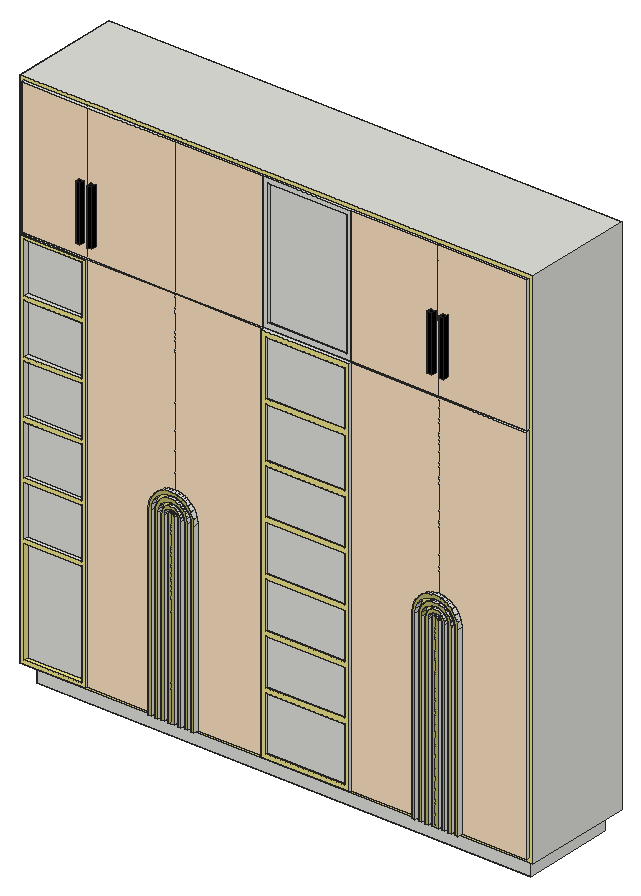
# SketchUp Ruby script. Lengths in inches.
U = 1.inch
M = Sketchup.active_model
def pt(a) = Geom::Point3d.new(a.map { |v| v * U })
def face(e, loops, mat)
  f = e.add_face(loops[0].map { |a| pt(a) })
  loops[1..].each { |l| e.add_face(l.map { |a| pt(a) }).erase! }
  f.material = f.back_material = mat if mat
  f
end
# faces: each face lists its corners as indices into pts; further lists are holes
def faces(e, pts, list, mat = nil) = list.each { |f| face(e, (f[0].is_a?(Array) ? f : [f]).map { |l| l.map { |i| pts[i] } }, mat) }
# xy, xz, yz: faces in a plane at the given z, y or x. An outline is a flat list of corners, or four numbers for a rectangle; further outlines are holes
def ring(l) = l.size == 4 ? [[l[0], l[1]], [l[2], l[1]], [l[2], l[3]], [l[0], l[3]]] : l.each_slice(2).to_a
def flat(e, list, mat, &to3) = list.each { |f| face(e, (f[0].is_a?(Array) ? f : [f]).map { |l| ring(l).map { |u, v| to3.(u, v) } }, mat) }
def xy(e, z, list, mat = nil) = flat(e, list, mat) { |x, y| [x, y, z] }
def xz(e, y, list, mat = nil) = flat(e, list, mat) { |x, z| [x, y, z] }
def yz(e, x, list, mat = nil) = flat(e, list, mat) { |y, z| [x, y, z] }
def lines(e, pts, list) = list.each { |a, b| e.add_line(pt(pts[a]), pt(pts[b])) }
# prism: a flat outline (further loops are holes) pulled along v
def prism(e, loops, v, mat = nil)
  f = face(e, loops, mat); d = Geom::Vector3d.new(v.map { |x| x * U })
  f.pushpull(f.normal.samedirection?(d) ? d.length : -d.length)
end
def box(e, o, s, mat = nil) = prism(e, [[o, [o[0] + s[0], o[1], o[2]], [o[0] + s[0], o[1] + s[1], o[2]], [o[0], o[1] + s[1], o[2]]]], [0, 0, s[2]], mat)
def at(x, y, z, deg = 0) = Geom::Transformation.translation(pt([x, y, z])) * Geom::Transformation.rotation(ORIGIN, Z_AXIS, deg.degrees)
def axes(o, x, y, z) = Geom::Transformation.new([*x, 0, *y, 0, *z, 0, *pt(o).to_a, 1])
def part(name) = M.definitions.add(name)
# library, detail: a bought-in or finely detailed component or shape, given as its bounding box
def library(name, o, s) = part(name).tap { |d| box(d.entities, o, s) }
def detail(e, o, s) = box(e.add_group.entities, o, s)
def put(e, d, t, mat = nil) = e.add_instance(d, t).tap { |i| i.material = mat if mat }
def group(e, t, mat = nil) = e.add_group.tap { |g| g.transformation = t; g.material = mat if mat }.entities
root = M.entities
M.materials.add("[0012_Bisque]").color = [255, 228, 196]
M.materials.add("[0047_Khaki]").color = [240, 230, 140]
M.materials.add("[0057_DarkKhaki]").color = [189, 183, 107]
M.materials.add("[0137_Black]").color = [0, 0, 0]
xy(root,-4,[[2,3.6,109,23.6]])
xy(root,0,[[[0,1.6,111,25.6],[2,3.6,109,23.6]]])
xy(root,0.8,[[0.8,0.6,15,1.6],[53,0.6,72,1.6]])
xy(root,0.8,[[29,0,29,1,15,1,15,1.6,34,1.6,34,0,33.29,0,33.29,1,32.57,1,32.57,0,31.86,0,31.86,1,31.14,1,31.14,0,30.43,0,30.43,1,29.71,1,29.71,0],[34,0,34,1.6,53,1.6,53,1,39,1,39,0,38.29,0,38.29,1,37.57,1,37.57,0,36.86,0,36.86,1,36.14,1,36.14,0,35.43,0,35.43,1,34.71,1,34.71,0],[86.1,0,86.1,1,72,1,72,1.6,91.1,1.6,91.1,0,90.39,0,90.39,1,89.67,1,89.67,0,88.96,0,88.96,1,88.24,1,88.24,0,87.53,0,87.53,1,86.8125,1,86.8125,0],[91.1,0,91.1,1.6,110.2,1.6,110.2,1,96.1,1,96.1,0,95.39,0,95.39,1,94.67,1,94.67,0,93.96,0,93.96,1,93.24,1,93.24,0,92.53,0,92.53,1,91.8125,1,91.8125,0]],"[0047_Khaki]")
xy(root,1.6,[[1.6,0.6,14.2,1.6]],"[0047_Khaki]")
xy(root,1.8,[[54,0.6,71,1]],"[0047_Khaki]")
xy(root,13.63,[[54,0.6,71,1]])
xy(root,14.63,[[54,0.6,71,1]],"[0047_Khaki]")
xy(root,24.2,[[1.6,0.6,14.2,1.6]])
xy(root,24.63,[[54,0.6,71,1]])
xy(root,25,[[1.6,0.6,14.2,1.6]])
xy(root,25.63,[[54,0.6,71,1]],"[0047_Khaki]")
xy(root,35.63,[[54,0.6,71,1]])
xy(root,36,[[1.6,0.6,14.2,1.6]])
xy(root,36.63,[[54,0.6,71,1]])
xy(root,36.8,[[1.6,0.6,14.2,1.6]])
xy(root,46.63,[[54,0.6,71,1]])
xy(root,47.63,[[54,0.6,71,1]])
xy(root,47.8,[[1.6,0.6,14.2,1.6]])
xy(root,48.6,[[1.6,0.6,14.2,1.6]])
xy(root,57.63,[[54,0.6,71,1]])
xy(root,58.63,[[54,0.6,71,1]])
xy(root,59.6,[[1.6,0.6,14.2,1.6]])
xy(root,60.4,[[1.6,0.6,14.2,1.6]])
xy(root,69.63,[[54,0.6,71,1]])
xy(root,70.63,[[54,0.6,71,1]])
xy(root,71.4,[[1.6,0.6,14.2,1.6]])
xy(root,72.2,[[1.6,0.6,14.2,1.6]])
xy(root,82.63,[[54,0.6,71,1]])
xy(root,83.2,[[1.6,0.6,14.2,1.6]])
xy(root,83.63,[[0.8,0.6,15,1],[53,0.6,72,0.6,72,1,110.2,1,110.2,1.6,0.8,1.6,0.8,1,53,1]])
xy(root,84,[[0.8,1,110.2,1.6],[53,1,72,1.125]])
xy(root,85,[[54,1.125,71,1.6]])
xy(root,86.77,[[13.29,0,14.29,1],[15.79,0,16.79,1]],"[0137_Black]")
xy(root,88.27,[[89.41,0,90.41,1],[91.97,0,92.97,1]],"[0137_Black]")
xy(root,98.77,[[13.29,0,14.29,1],[15.79,0,16.79,1]],"[0137_Black]")
xy(root,100.27,[[89.41,0,90.41,1],[91.97,0,92.97,1]],"[0137_Black]")
xy(root,112.2,[[54,1.125,71,1.6]])
xy(root,113.2,[[0.8,1,15,1.6],[15,1,34,1.6],[34,1,53,1.6],[72,1,91,1.6],[91,1,110.2,1.6],
  [53,1.125,72,1.6]])
xy(root,114,[[0,1.6,111,25.6]])
xz(root,0,[[29,0.8,29.71,0.8,29.71,40.8,29.86,41.91,30.29,42.94,30.43,43.125,30.97,43.83,31.14,43.96,31.86,44.51,32.57,44.81,32.89,44.94,33.29,44.99,34,45.09,34.71,44.99,35.11,44.94,35.43,44.81,36.14,44.51,36.86,43.96,37.03,43.83,37.57,43.125,37.71,42.94,38.14,41.91,38.29,40.8,38.29,0.8,39,0.8,39,40.8,38.83,42.09,38.33,43.3,38.29,43.36,37.57,44.29,37.54,44.34,36.86,44.86,36.5,45.13,36.14,45.28,35.43,45.57,35.29,45.63,34.71,45.71,34,45.8,33.29,45.71,32.71,45.63,32.57,45.57,31.86,45.28,31.5,45.13,31.14,44.86,30.46,44.34,30.43,44.29,29.71,43.36,29.67,43.3,29.17,42.09,29,40.8],[30.43,0.8,31.14,0.8,31.14,40.8,31.24,41.54,31.53,42.23,31.86,42.66,31.98,42.82,32.57,43.27,33.26,43.56,33.29,43.5625,34,43.66,34.71,43.5625,34.74,43.56,35.43,43.27,36.02,42.82,36.14,42.66,36.47,42.23,36.76,41.54,36.86,40.8,36.86,0.8,37.57,0.8,37.57,40.8,37.45,41.72,37.09,42.59,36.86,42.89,36.53,43.33,36.14,43.62,35.79,43.89,35.43,44.04,34.92,44.25,34.71,44.28,34,44.37,33.29,44.28,33.08,44.25,32.57,44.04,32.21,43.89,31.86,43.62,31.47,43.33,31.14,42.89,30.91,42.59,30.55,41.72,30.43,40.8],[31.86,0.8,32.57,0.8,32.57,40.8,32.59,41.2,32.72,41.57,32.94,41.9,33.25,42.15,33.29,42.17,33.61,42.31,34,42.36,34.39,42.31,34.71,42.17,34.75,42.15,35.06,41.9,35.28,41.57,35.41,41.2,35.43,40.8,35.43,0.8,36.14,0.8,36.14,40.8,36.07,41.35,35.86,41.87,35.52,42.32,35.43,42.38,35.07,42.66,34.71,42.8,34.55,42.87,34,42.94,33.45,42.87,33.29,42.8,32.93,42.66,32.57,42.38,32.48,42.32,32.14,41.87,31.93,41.35,31.86,40.8],[33.29,0.8,34,0.8,34,41.8,33.83,41.78,33.67,41.72,33.52,41.62,33.41,41.49,33.33,41.34,33.29,41.17],[34,0.8,34.71,0.8,34.71,41.17,34.67,41.34,34.59,41.49,34.48,41.62,34.33,41.72,34.17,41.78,34,41.8],
  [86.1,0.8,86.8125,0.8,86.8125,40.8,86.96,41.91,87.39,42.94,87.53,43.125,88.07,43.83,88.24,43.96,88.96,44.51,89.67,44.81,89.99,44.94,90.39,44.99,91.1,45.09,91.8125,44.99,92.21,44.94,92.53,44.81,93.24,44.51,93.96,43.96,94.13,43.83,94.67,43.125,94.8125,42.94,95.24,41.91,95.39,40.8,95.39,0.8,96.1,0.8,96.1,40.8,95.93,42.09,95.43,43.3,95.39,43.36,94.67,44.29,94.64,44.34,93.96,44.86,93.6,45.13,93.24,45.28,92.53,45.57,92.39,45.63,91.8125,45.71,91.1,45.8,90.39,45.71,89.81,45.63,89.67,45.57,88.96,45.28,88.6,45.13,88.24,44.86,87.5625,44.34,87.53,44.29,86.8125,43.36,86.77,43.3,86.27,42.09,86.1,40.8],[87.53,0.8,88.24,0.8,88.24,40.8,88.34,41.54,88.625,42.23,88.96,42.66,89.08,42.82,89.67,43.27,90.36,43.56,90.39,43.5625,91.1,43.66,91.8125,43.5625,91.84,43.56,92.53,43.27,93.12,42.82,93.24,42.66,93.57,42.23,93.86,41.54,93.96,40.8,93.96,0.8,94.67,0.8,94.67,40.8,94.55,41.72,94.19,42.59,93.96,42.89,93.625,43.33,93.24,43.62,92.89,43.89,92.53,44.04,92.02,44.25,91.8125,44.28,91.1,44.37,90.39,44.28,90.18,44.25,89.67,44.04,89.3125,43.89,88.96,43.62,88.57,43.33,88.24,42.89,88.01,42.59,87.65,41.72,87.53,40.8],[88.96,0.8,89.67,0.8,89.67,40.8,89.69,41.2,89.82,41.57,90.04,41.9,90.35,42.15,90.39,42.17,90.71,42.31,91.1,42.36,91.49,42.31,91.8125,42.17,91.85,42.15,92.16,41.9,92.38,41.57,92.51,41.2,92.53,40.8,92.53,0.8,93.24,0.8,93.24,40.8,93.17,41.35,92.96,41.87,92.62,42.32,92.53,42.38,92.17,42.66,91.8125,42.8,91.65,42.87,91.1,42.94,90.55,42.87,90.39,42.8,90.03,42.66,89.67,42.38,89.58,42.32,89.24,41.87,89.03,41.35,88.96,40.8],[90.39,0.8,91.1,0.8,91.1,41.8,90.93,41.78,90.77,41.72,90.625,41.62,90.51,41.49,90.43,41.34,90.39,41.17],[91.1,0.8,91.8125,0.8,91.8125,41.17,91.77,41.34,91.69,41.49,91.58,41.62,91.43,41.72,91.27,41.78,91.1,41.8]],"[0057_DarkKhaki]")
xz(root,0,[[13.29,86.77,14.29,98.77],[15.79,86.77,16.79,98.77],[89.41,88.27,90.41,100.27],[91.97,88.27,92.97,100.27]],"[0137_Black]")
xz(root,0.6,[[[0.8,0.8,15,83.63],[1.6,1.6,14.2,24.2],[1.6,72.2,14.2,83.2],[1.6,60.4,14.2,71.4],[1.6,48.6,14.2,59.6],[1.6,36.8,14.2,47.8],[1.6,25,14.2,36]],[[53,0.8,72,83.63],[54,70.63,71,82.63],[54,1.8,71,13.63],[54,58.63,71,69.63],[54,47.63,71,57.63],[54,36.63,71,46.63],[54,25.63,71,35.63],[54,14.63,71,24.63]]],"[0047_Khaki]")
xz(root,1,[[54,1.8,71,13.63],[54,14.63,71,24.63],[54,25.63,71,35.63],[54,36.63,71,46.63],[54,47.63,71,57.63],
  [54,58.63,71,69.63],[54,70.63,71,82.63],[89.41,88.27,90.41,100.27],[91.97,88.27,92.97,100.27]])
xz(root,1,[[15,0.8,29,0.8,29,40.8,29.17,42.09,29.67,43.3,29.71,43.36,30.43,44.29,30.46,44.34,31.14,44.86,31.5,45.13,31.86,45.28,32.57,45.57,32.71,45.63,33.29,45.71,34,45.8,34,83.63,15,83.63],[39,0.8,53,0.8,53,83.63,34,83.63,34,45.8,34.71,45.71,35.29,45.63,35.43,45.57,36.14,45.28,36.5,45.13,36.86,44.86,37.54,44.34,37.57,44.29,38.29,43.36,38.33,43.3,38.83,42.09,39,40.8],[72,0.8,86.1,0.8,86.1,40.8,86.27,42.09,86.77,43.3,86.8125,43.36,87.53,44.29,87.5625,44.34,88.24,44.86,88.6,45.13,88.96,45.28,89.67,45.57,89.81,45.63,90.39,45.71,91.1,45.8,91.1,83.63,72,83.63],[96.1,0.8,110.2,0.8,110.2,83.63,91.1,83.63,91.1,45.8,91.8125,45.71,92.39,45.63,92.53,45.57,93.24,45.28,93.6,45.13,93.96,44.86,94.64,44.34,94.67,44.29,95.39,43.36,95.43,43.3,95.93,42.09,96.1,40.8],[[0.8,84,15,113.2],[13.29,86.77,14.29,98.77]],
  [[15,84,34,113.2],[15.79,86.77,16.79,98.77]],[34,84,53,113.2],[[72,84,91.1,84,91,113.2,72,113.2],[89.41,88.27,90.41,100.27]],[[91.1,84,110.2,84,110.2,113.2,91,113.2],[91.97,88.27,92.97,100.27]],[13.29,86.77,14.29,98.77],
  [15.79,86.77,16.79,98.77]],"[0012_Bisque]")
xz(root,1,[[29.71,0.8,30.43,0.8,30.43,40.8,30.55,41.72,30.91,42.59,31.14,42.89,31.47,43.33,31.86,43.62,32.21,43.89,32.57,44.04,33.08,44.25,33.29,44.28,34,44.37,34.71,44.28,34.92,44.25,35.43,44.04,35.79,43.89,36.14,43.62,36.53,43.33,36.86,42.89,37.09,42.59,37.45,41.72,37.57,40.8,37.57,0.8,38.29,0.8,38.29,40.8,38.14,41.91,37.71,42.94,37.57,43.125,37.03,43.83,36.86,43.96,36.14,44.51,35.43,44.81,35.11,44.94,34.71,44.99,34,45.09,33.29,44.99,32.89,44.94,32.57,44.81,31.86,44.51,31.14,43.96,30.97,43.83,30.43,43.125,30.29,42.94,29.86,41.91,29.71,40.8],[31.14,0.8,31.86,0.8,31.86,40.8,31.93,41.35,32.14,41.87,32.48,42.32,32.57,42.38,32.93,42.66,33.29,42.8,33.45,42.87,34,42.94,34.55,42.87,34.71,42.8,35.07,42.66,35.43,42.38,35.52,42.32,35.86,41.87,36.07,41.35,36.14,40.8,36.14,0.8,36.86,0.8,36.86,40.8,36.76,41.54,36.47,42.23,36.14,42.66,36.02,42.82,35.43,43.27,34.74,43.56,34.71,43.5625,34,43.66,33.29,43.5625,33.26,43.56,32.57,43.27,31.98,42.82,31.86,42.66,31.53,42.23,31.24,41.54,31.14,40.8],[32.57,0.8,33.29,0.8,33.29,41.17,33.33,41.34,33.41,41.49,33.52,41.62,33.67,41.72,33.83,41.78,34,41.8,34.17,41.78,34.33,41.72,34.48,41.62,34.59,41.49,34.67,41.34,34.71,41.17,34.71,0.8,35.43,0.8,35.43,40.8,35.41,41.2,35.28,41.57,35.06,41.9,34.75,42.15,34.71,42.17,34.39,42.31,34,42.36,33.61,42.31,33.29,42.17,33.25,42.15,32.94,41.9,32.72,41.57,32.59,41.2,32.57,40.8],[86.8125,0.8,87.53,0.8,87.53,40.8,87.65,41.72,88.01,42.59,88.24,42.89,88.57,43.33,88.96,43.62,89.3125,43.89,89.67,44.04,90.18,44.25,90.39,44.28,91.1,44.37,91.8125,44.28,92.02,44.25,92.53,44.04,92.89,43.89,93.24,43.62,93.625,43.33,93.96,42.89,94.19,42.59,94.55,41.72,94.67,40.8,94.67,0.8,95.39,0.8,95.39,40.8,95.24,41.91,94.8125,42.94,94.67,43.125,94.13,43.83,93.96,43.96,93.24,44.51,92.53,44.81,92.21,44.94,91.8125,44.99,91.1,45.09,90.39,44.99,89.99,44.94,89.67,44.81,88.96,44.51,88.24,43.96,88.07,43.83,87.53,43.125,87.39,42.94,86.96,41.91,86.8125,40.8],[88.24,0.8,88.96,0.8,88.96,40.8,89.03,41.35,89.24,41.87,89.58,42.32,89.67,42.38,90.03,42.66,90.39,42.8,90.55,42.87,91.1,42.94,91.65,42.87,91.8125,42.8,92.17,42.66,92.53,42.38,92.62,42.32,92.96,41.87,93.17,41.35,93.24,40.8,93.24,0.8,93.96,0.8,93.96,40.8,93.86,41.54,93.57,42.23,93.24,42.66,93.12,42.82,92.53,43.27,91.84,43.56,91.8125,43.5625,91.1,43.66,90.39,43.5625,90.36,43.56,89.67,43.27,89.08,42.82,88.96,42.66,88.625,42.23,88.34,41.54,88.24,40.8],
  [89.67,0.8,90.39,0.8,90.39,41.17,90.43,41.34,90.51,41.49,90.625,41.62,90.77,41.72,90.93,41.78,91.1,41.8,91.27,41.78,91.43,41.72,91.58,41.62,91.69,41.49,91.77,41.34,91.8125,41.17,91.8125,0.8,92.53,0.8,92.53,40.8,92.51,41.2,92.38,41.57,92.16,41.9,91.85,42.15,91.8125,42.17,91.49,42.31,91.1,42.36,90.71,42.31,90.39,42.17,90.35,42.15,90.04,41.9,89.82,41.57,89.69,41.2,89.67,40.8]],"[0047_Khaki]")
xz(root,1.125,[[[53,84,72,113.2],[54,85,71,112.2]]])
xz(root,1.6,[[1.6,1.6,14.2,24.2],[1.6,25,14.2,36],[1.6,36.8,14.2,47.8],[1.6,48.6,14.2,59.6],[1.6,60.4,14.2,71.4],
  [1.6,72.2,14.2,83.2],[54,85,71,112.2]])
xz(root,1.6,[[[0,0,111,0,111,114,91,114,91,113.2,110.2,113.2,110.2,84,0.8,84,0.8,113.2,91,113.2,91,114,0,114],[0.8,0.8,110.2,83.63]]],"[0047_Khaki]")
xz(root,3.6,[[2,-4,109,0]])
xz(root,23.6,[[2,-4,109,0]])
xz(root,25.6,[[0,0,111,114]])
yz(root,0,[[1.6,0,25.6,114]])
yz(root,0.8,[[0.6,0.8,1.6,83.63],[1,84,1.6,113.2]])
yz(root,1.6,[[0.6,25,1.6,36],[0.6,36.8,1.6,47.8],[0.6,48.6,1.6,59.6],[0.6,60.4,1.6,71.4],[0.6,72.2,1.6,83.2]])
yz(root,1.6,[[0.6,1.6,1.6,24.2]],"[0047_Khaki]")
yz(root,2,[[3.6,-4,23.6,0]])
yz(root,13.29,[[0,86.77,1,98.77]],"[0137_Black]")
yz(root,14.2,[[0.6,25,1.6,36],[0.6,36.8,1.6,47.8],[0.6,48.6,1.6,59.6],[0.6,60.4,1.6,71.4],[0.6,72.2,1.6,83.2]])
yz(root,14.2,[[0.6,1.6,1.6,24.2]],"[0047_Khaki]")
yz(root,14.29,[[0,86.77,1,98.77]],"[0137_Black]")
yz(root,15,[[0.6,0.8,1,83.63]])
yz(root,15.79,[[0,86.77,1,98.77]],"[0137_Black]")
yz(root,16.79,[[0,86.77,1,98.77]],"[0137_Black]")
yz(root,29,[[0,0.8,1,40.8]])
yz(root,29.71,[[0,0.8,1,40.8]])
yz(root,30.43,[[0,0.8,1,40.8]])
yz(root,31.14,[[0,0.8,1,40.8]])
yz(root,31.86,[[0,0.8,1,40.8]])
yz(root,32.57,[[0,0.8,1,40.8]])
yz(root,33.29,[[0,0.8,1,41.17]])
yz(root,34.71,[[0,0.8,1,41.17]])
yz(root,35.43,[[0,0.8,1,40.8]])
yz(root,36.14,[[0,0.8,1,40.8]])
yz(root,36.86,[[0,0.8,1,40.8]])
yz(root,37.57,[[0,0.8,1,40.8]])
yz(root,38.29,[[0,0.8,1,40.8]])
yz(root,39,[[0,0.8,1,40.8]])
yz(root,53,[[0.6,0.8,1,83.63],[1,84,1.125,113.2]])
yz(root,54,[[0.6,1.8,1,13.63],[0.6,14.63,1,24.63],[0.6,25.63,1,35.63],[0.6,36.63,1,46.63],[0.6,47.63,1,57.63],
  [0.6,58.63,1,69.63],[0.6,70.63,1,82.63],[1.125,85,1.6,112.2]])
yz(root,71,[[0.6,36.63,1,46.63],[0.6,47.63,1,57.63],[0.6,58.63,1,69.63],[0.6,70.63,1,82.63],[1.125,85,1.6,112.2]])
yz(root,71,[[0.6,1.8,1,13.63],[0.6,14.63,1,24.63],[0.6,25.63,1,35.63]],"[0047_Khaki]")
yz(root,72,[[0.6,0.8,1,83.63],[1,84,1.125,113.2]])
yz(root,86.1,[[0,0.8,1,40.8]])
yz(root,86.8125,[[0,0.8,1,40.8]])
yz(root,87.53,[[0,0.8,1,40.8]])
yz(root,88.24,[[0,0.8,1,40.8]])
yz(root,88.96,[[0,0.8,1,40.8]])
yz(root,89.41,[[0,88.27,1,100.27]],"[0137_Black]")
yz(root,89.67,[[0,0.8,1,40.8]])
yz(root,90.39,[[0,0.8,1,41.17]])
yz(root,90.41,[[0,88.27,1,100.27]],"[0137_Black]")
yz(root,91.8125,[[0,0.8,1,41.17]])
yz(root,91.97,[[0,88.27,1,100.27]],"[0137_Black]")
yz(root,92.53,[[0,0.8,1,40.8]])
yz(root,92.97,[[0,88.27,1,100.27]],"[0137_Black]")
yz(root,93.24,[[0,0.8,1,40.8]])
yz(root,93.96,[[0,0.8,1,40.8]])
yz(root,94.67,[[0,0.8,1,40.8]])
yz(root,95.39,[[0,0.8,1,40.8]])
yz(root,96.1,[[0,0.8,1,40.8]])
yz(root,109,[[3.6,-4,23.6,0]])
yz(root,110.2,[[1,0.8,1.6,83.63],[1,84,1.6,113.2]])
yz(root,111,[[1.6,0,25.6,114]])
p = [[29.17,1,42.09],[29,1,40.8],[29,0,40.8],[29.17,0,42.09],[29.71,1,40.8],[29.86,1,41.91],
  [29.86,0,41.91],[29.71,0,40.8],[30.55,1,41.72],[30.43,1,40.8],[30.43,0,40.8],[30.55,0,41.72],
  [31.14,1,40.8],[31.24,1,41.54],[31.24,0,41.54],[31.14,0,40.8],[31.93,1,41.35],[31.86,1,40.8],
  [31.86,0,40.8],[31.93,0,41.35],[32.57,1,40.8],[32.59,1,41.2],[32.59,0,41.2],[32.57,0,40.8],
  [35.41,1,41.2],[35.43,1,40.8],[35.43,0,40.8],[35.41,0,41.2],[36.14,1,40.8],[36.07,1,41.35],
  [36.07,0,41.35],[36.14,0,40.8],[36.76,1,41.54],[36.86,1,40.8],[36.86,0,40.8],[36.76,0,41.54],
  [37.57,1,40.8],[37.45,1,41.72],[37.45,0,41.72],[37.57,0,40.8],[38.14,1,41.91],[38.29,1,40.8],
  [38.29,0,40.8],[38.14,0,41.91],[39,1,40.8],[38.83,1,42.09],[38.83,0,42.09],[39,0,40.8],
  [86.27,1,42.09],[86.1,1,40.8],[86.1,0,40.8],[86.27,0,42.09],[86.8125,1,40.8],[86.96,1,41.91],
  [86.96,0,41.91],[86.8125,0,40.8],[87.65,1,41.72],[87.53,1,40.8],[87.53,0,40.8],[87.65,0,41.72],
  [88.24,1,40.8],[88.34,1,41.54],[88.34,0,41.54],[88.24,0,40.8],[89.03,1,41.35],[88.96,1,40.8],
  [88.96,0,40.8],[89.03,0,41.35],[89.67,1,40.8],[89.69,1,41.2],[89.69,0,41.2],[89.67,0,40.8],
  [92.51,1,41.2],[92.53,1,40.8],[92.53,0,40.8],[92.51,0,41.2],[93.24,1,40.8],[93.17,1,41.35],
  [93.17,0,41.35],[93.24,0,40.8],[93.86,1,41.54],[93.96,1,40.8],[93.96,0,40.8],[93.86,0,41.54],
  [94.67,1,40.8],[94.55,1,41.72],[94.55,0,41.72],[94.67,0,40.8],[95.24,1,41.91],[95.39,1,40.8],
  [95.39,0,40.8],[95.24,0,41.91],[96.1,1,40.8],[95.93,1,42.09],[95.93,0,42.09],[96.1,0,40.8],
  [32.72,1,41.57],[32.72,0,41.57],[33.33,1,41.34],[33.29,1,41.17],[33.29,0,41.17],[33.33,0,41.34],
  [34.71,1,41.17],[34.67,1,41.34],[34.67,0,41.34],[34.71,0,41.17],[35.28,1,41.57],[35.28,0,41.57],
  [89.82,1,41.57],[89.82,0,41.57],[90.43,1,41.34],[90.39,1,41.17],[90.39,0,41.17],[90.43,0,41.34],
  [91.8125,1,41.17],[91.77,1,41.34],[91.77,0,41.34],[91.8125,0,41.17],[92.38,1,41.57],[92.38,0,41.57],
  [33.41,1,41.49],[33.41,0,41.49],[34.59,1,41.49],[34.59,0,41.49],[90.51,1,41.49],[90.51,0,41.49],
  [91.69,1,41.49],[91.69,0,41.49],[32.14,1,41.87],[32.14,0,41.87],[35.86,1,41.87],[35.86,0,41.87],
  [89.24,1,41.87],[89.24,0,41.87],[92.96,1,41.87],[92.96,0,41.87],[31.53,1,42.23],[31.53,0,42.23],
  [33.52,1,41.62],[33.52,0,41.62],[34.48,1,41.62],[34.48,0,41.62],[36.47,1,42.23],[36.47,0,42.23],
  [88.625,1,42.23],[88.625,0,42.23],[90.625,1,41.62],[90.625,0,41.62],[91.58,1,41.62],[91.58,0,41.62],
  [93.57,1,42.23],[93.57,0,42.23],[32.94,1,41.9],[32.94,0,41.9],[33.67,1,41.72],[33.67,0,41.72],
  [34.33,1,41.72],[34.33,0,41.72],[35.06,1,41.9],[35.06,0,41.9],[90.04,1,41.9],[90.04,0,41.9],
  [90.77,1,41.72],[90.77,0,41.72],[91.43,1,41.72],[91.43,0,41.72],[92.16,1,41.9],[92.16,0,41.9],
  [30.91,1,42.59],[30.91,0,42.59],[33.83,1,41.78],[33.83,0,41.78],[34.17,1,41.78],[34.17,0,41.78],
  [37.09,1,42.59],[37.09,0,42.59],[88.01,1,42.59],[88.01,0,42.59],[90.93,1,41.78],[90.93,0,41.78],
  [91.27,1,41.78],[91.27,0,41.78],[94.19,1,42.59],[94.19,0,42.59],[34,1,41.8],[34,0,41.8],
  [91.1,1,41.8],[91.1,0,41.8],[30.29,1,42.94],[30.29,0,42.94],[32.48,1,42.32],[32.48,0,42.32],
  [33.25,1,42.15],[33.25,0,42.15],[34.75,1,42.15],[34.75,0,42.15],[35.52,1,42.32],[35.52,0,42.32],
  [37.71,1,42.94],[37.71,0,42.94],[87.39,1,42.94],[87.39,0,42.94],[89.58,1,42.32],[89.58,0,42.32],
  [90.35,1,42.15],[90.35,0,42.15],[91.85,1,42.15],[91.85,0,42.15],[92.62,1,42.32],[92.62,0,42.32],
  [94.8125,1,42.94],[94.8125,0,42.94],[29.67,1,43.3],[29.67,0,43.3],[33.29,1,42.17],[33.29,0,42.17],
  [34.71,1,42.17],[34.71,0,42.17],[38.33,1,43.3],[38.33,0,43.3],[86.77,1,43.3],[86.77,0,43.3],
  [90.39,1,42.17],[90.39,0,42.17],[91.8125,1,42.17],[91.8125,0,42.17],[95.43,1,43.3],[95.43,0,43.3],
  [31.86,1,42.66],[31.86,0,42.66],[33.61,1,42.31],[33.61,0,42.31],[34.39,1,42.31],[34.39,0,42.31],
  [36.14,1,42.66],[36.14,0,42.66],[88.96,1,42.66],[88.96,0,42.66],[90.71,1,42.31],[90.71,0,42.31],
  [91.49,1,42.31],[91.49,0,42.31],[93.24,1,42.66],[93.24,0,42.66],[32.57,1,42.38],[32.57,0,42.38],
  [34,1,42.36],[34,0,42.36],[35.43,1,42.38],[35.43,0,42.38],[89.67,1,42.38],[89.67,0,42.38],
  [91.1,1,42.36],[91.1,0,42.36],[92.53,1,42.38],[92.53,0,42.38],[32.93,1,42.66],[32.93,0,42.66],
  [35.07,1,42.66],[35.07,0,42.66],[90.03,1,42.66],[90.03,0,42.66],[92.17,1,42.66],[92.17,0,42.66],
  [31.14,1,42.89],[31.14,0,42.89],[36.86,1,42.89],[36.86,0,42.89],[88.24,1,42.89],[88.24,0,42.89],
  [93.96,1,42.89],[93.96,0,42.89],[31.98,1,42.82],[31.98,0,42.82],[33.29,1,42.8],[33.29,0,42.8],
  [34.71,1,42.8],[34.71,0,42.8],[36.02,1,42.82],[36.02,0,42.82],[89.08,1,42.82],[89.08,0,42.82],
  [90.39,1,42.8],[90.39,0,42.8],[91.8125,1,42.8],[91.8125,0,42.8],[93.12,1,42.82],[93.12,0,42.82],
  [32.57,1,43.27],[32.57,0,43.27],[33.45,1,42.87],[33.45,0,42.87],[34.55,1,42.87],[34.55,0,42.87],
  [35.43,1,43.27],[35.43,0,43.27],[89.67,1,43.27],[89.67,0,43.27],[90.55,1,42.87],[90.55,0,42.87],
  [91.65,1,42.87],[91.65,0,42.87],[92.53,1,43.27],[92.53,0,43.27],[30.43,1,43.125],[30.43,0,43.125],
  [31.47,1,43.33],[31.47,0,43.33],[34,1,42.94],[34,0,42.94],[36.53,1,43.33],[36.53,0,43.33],
  [37.57,1,43.125],[37.57,0,43.125],[87.53,1,43.125],[87.53,0,43.125],[88.57,1,43.33],[88.57,0,43.33],
  [91.1,1,42.94],[91.1,0,42.94],[93.625,1,43.33],[93.625,0,43.33],[94.67,1,43.125],[94.67,0,43.125],
  [30.97,1,43.83],[30.97,0,43.83],[37.03,1,43.83],[37.03,0,43.83],[88.07,1,43.83],[88.07,0,43.83],
  [94.13,1,43.83],[94.13,0,43.83],[29.71,1,43.36],[29.71,0,43.36],[31.86,1,43.62],[31.86,0,43.62],
  [33.26,1,43.56],[33.26,0,43.56],[34.74,1,43.56],[34.74,0,43.56],[36.14,1,43.62],[36.14,0,43.62],
  [38.29,1,43.36],[38.29,0,43.36],[86.8125,1,43.36],[86.8125,0,43.36],[88.96,1,43.62],[88.96,0,43.62],
  [90.36,1,43.56],[90.36,0,43.56],[91.84,1,43.56],[91.84,0,43.56],[93.24,1,43.62],[93.24,0,43.62],
  [95.39,1,43.36],[95.39,0,43.36],[30.43,1,44.29],[30.43,0,44.29],[37.57,1,44.29],[37.57,0,44.29],
  [87.53,1,44.29],[87.53,0,44.29],[94.67,1,44.29],[94.67,0,44.29],[32.21,1,43.89],[32.21,0,43.89],
  [33.29,1,43.5625],[33.29,0,43.5625],[34,1,43.66],[34,0,43.66],[34.71,1,43.5625],[34.71,0,43.5625],
  [35.79,1,43.89],[35.79,0,43.89],[89.3125,1,43.89],[89.3125,0,43.89],[90.39,1,43.5625],[90.39,0,43.5625],
  [91.1,1,43.66],[91.1,0,43.66],[91.8125,1,43.5625],[91.8125,0,43.5625],[92.89,1,43.89],[92.89,0,43.89],
  [31.14,1,43.96],[31.14,0,43.96],[36.86,1,43.96],[36.86,0,43.96],[88.24,1,43.96],[88.24,0,43.96],
  [93.96,1,43.96],[93.96,0,43.96],[32.57,1,44.04],[32.57,0,44.04],[35.43,1,44.04],[35.43,0,44.04],
  [89.67,1,44.04],[89.67,0,44.04],[92.53,1,44.04],[92.53,0,44.04],[31.86,1,44.51],[31.86,0,44.51],
  [33.08,1,44.25],[33.08,0,44.25],[34.92,1,44.25],[34.92,0,44.25],[36.14,1,44.51],[36.14,0,44.51],
  [88.96,1,44.51],[88.96,0,44.51],[90.18,1,44.25],[90.18,0,44.25],[92.02,1,44.25],[92.02,0,44.25],
  [93.24,1,44.51],[93.24,0,44.51],[33.29,1,44.28],[33.29,0,44.28],[34.71,1,44.28],[34.71,0,44.28],
  [90.39,1,44.28],[90.39,0,44.28],[91.8125,1,44.28],[91.8125,0,44.28],[30.46,1,44.34],[30.46,0,44.34],
  [31.14,1,44.86],[31.14,0,44.86],[34,1,44.37],[34,0,44.37],[37.54,1,44.34],[36.86,1,44.86],
  [36.86,0,44.86],[37.54,0,44.34],[87.5625,1,44.34],[87.5625,0,44.34],[88.24,1,44.86],[88.24,0,44.86],
  [91.1,1,44.37],[91.1,0,44.37],[94.64,1,44.34],[93.96,1,44.86],[93.96,0,44.86],[94.64,0,44.34],
  [32.57,1,44.81],[32.57,0,44.81],[35.43,1,44.81],[35.43,0,44.81],[89.67,1,44.81],[89.67,0,44.81],
  [92.53,1,44.81],[92.53,0,44.81],[32.89,1,44.94],[32.89,0,44.94],[35.11,1,44.94],[35.11,0,44.94],
  [89.99,1,44.94],[89.99,0,44.94],[92.21,1,44.94],[92.21,0,44.94],[31.5,1,45.13],[31.5,0,45.13],
  [33.29,1,44.99],[33.29,0,44.99],[34.71,1,44.99],[34.71,0,44.99],[36.5,1,45.13],[36.5,0,45.13],
  [88.6,1,45.13],[88.6,0,45.13],[90.39,1,44.99],[90.39,0,44.99],[91.8125,1,44.99],[91.8125,0,44.99],
  [93.6,1,45.13],[93.6,0,45.13],[34,1,45.09],[34,0,45.09],[91.1,1,45.09],[91.1,0,45.09],
  [31.86,1,45.28],[31.86,0,45.28],[36.14,1,45.28],[36.14,0,45.28],[88.96,1,45.28],[88.96,0,45.28],
  [93.24,1,45.28],[93.24,0,45.28],[32.57,1,45.57],[32.57,0,45.57],[35.43,1,45.57],[35.43,0,45.57],
  [89.67,1,45.57],[89.67,0,45.57],[92.53,1,45.57],[92.53,0,45.57],[32.71,1,45.63],[32.71,0,45.63],
  [33.29,1,45.71],[33.29,0,45.71],[35.29,1,45.63],[34.71,1,45.71],[34.71,0,45.71],[35.29,0,45.63],
  [89.81,1,45.63],[89.81,0,45.63],[90.39,1,45.71],[90.39,0,45.71],[92.39,1,45.63],[91.8125,1,45.71],
  [91.8125,0,45.71],[92.39,0,45.63],[34,1,45.8],[34,0,45.8],[91.1,1,45.8],[91.1,0,45.8],
  [34,0,41.84]]
faces(root,p,[[0,1,2,3],[4,5,6,7],[8,9,10,11],[12,13,14,15],[16,17,18,19],[20,21,22,23],[24,25,26,27],[28,29,30,31],
  [32,33,34,35],[36,37,38,39],[40,41,42,43],[44,45,46,47],[48,49,50,51],[52,53,54,55],[56,57,58,59],[64,65,66,67],
  [68,69,70,71],[72,73,74,75],[76,77,78,79],[84,85,86,87],[88,89,90,91],[92,93,94,95],[21,96,97,22],[98,99,100,101],
  [102,103,104,105],[106,24,27,107],[69,108,109,70],[110,111,112,113],[114,115,116,117],[118,72,75,119],[120,98,101,121],[103,122,123,104],
  [124,110,113,125],[115,126,127,116],[128,16,19,129],[29,130,131,30],[132,64,67,133],[77,134,135,78],[13,136,137,14],[138,120,121,139],
  [122,140,141,123],[142,32,35,143],[146,124,125,147],[126,148,149,127],[96,152,153,97],[154,138,139,155],[140,156,157,141],[158,106,107,159],
  [108,160,161,109],[162,146,147,163],[148,164,165,149],[166,118,119,167],[168,8,11,169],[170,154,155,171],[156,172,173,157],[37,174,175,38],
  [176,56,59,177],[178,162,163,179],[164,180,181,165],[85,182,183,86],[184,170,171,185],[172,184,185,173],[186,178,179,187],[180,186,187,181],
  [5,188,189,6],[190,128,129,191],[152,192,193,153],[194,158,159,195],[130,196,197,131],[198,40,43,199],[53,200,201,54],[202,132,133,203],
  [160,204,205,161],[206,166,167,207],[134,208,209,135],[210,88,91,211],[212,0,3,213],[192,214,215,193],[216,194,195,217],[45,218,219,46],
  [220,48,51,221],[204,222,223,205],[224,206,207,225],[93,226,227,94],[136,228,229,137],[214,230,231,215],[232,216,217,233],[234,142,143,235],
  [222,238,239,223],[240,224,225,241],[244,190,191,245],[230,246,247,231],[246,232,233,247],[196,248,249,197],[250,202,203,251],[238,252,253,239],
  [252,240,241,253],[208,254,255,209],[256,244,245,257],[248,258,259,249],[260,250,251,261],[254,262,263,255],[264,168,169,265],[174,266,267,175],
  [268,176,177,269],[182,270,271,183],[228,272,273,229],[274,256,257,275],[258,276,277,259],[278,234,235,279],[282,260,261,283],[262,284,285,263],
  [272,288,289,273],[290,274,275,291],[276,292,293,277],[294,278,279,295],[298,282,283,299],[284,300,301,285],[188,304,305,189],[306,264,265,307],
  [308,290,291,309],[292,308,309,293],[266,310,311,267],[312,198,199,313],[200,314,315,201],[316,268,269,317],[318,298,299,319],[300,318,319,301],
  [270,320,321,271],[322,210,211,323],[304,324,325,305],[326,312,313,327],[314,328,329,315],[330,322,323,331],[332,212,213,333],[334,306,307,335],
  [288,336,337,289],[338,294,295,339],[310,340,341,311],[218,342,343,219],[344,220,221,345],[346,316,317,347],[320,352,353,321],[226,354,355,227],
  [356,332,333,357],[342,358,359,343],[360,344,345,361],[354,362,363,355],[364,334,335,365],[336,366,367,337],[366,368,369,367],[368,370,371,369],
  [370,338,339,371],[340,372,373,341],[374,346,347,375],[352,382,383,353],[324,384,385,325],[386,326,327,387],[328,388,389,329],[390,330,331,391],
  [392,364,365,393],[372,394,395,373],[396,374,375,397],[382,398,399,383],[384,400,401,385],[402,392,393,403],[394,404,405,395],[406,386,387,407],
  [388,408,409,389],[410,396,397,411],[398,412,413,399],[414,390,391,415],[416,402,403,417],[404,418,419,405],[420,410,411,421],[412,422,423,413],
  [424,356,357,425],[426,424,425,427],[428,416,417,429],[418,428,429,419],[430,431,432,433],[358,430,433,359],[434,360,361,435],[436,434,435,437],
  [438,420,421,439],[422,438,439,423],[440,441,442,443],[362,440,443,363],[400,444,445,401],[446,406,407,447],[408,448,449,409],[450,414,415,451],
  [444,452,453,445],[454,446,447,455],[448,456,457,449],[458,450,451,459],[460,426,427,461],[452,462,463,453],[464,454,455,465],[431,466,467,432],
  [468,436,437,469],[456,470,471,457],[472,458,459,473],[441,474,475,442],[462,476,477,463],[476,464,465,477],[470,478,479,471],[478,472,473,479],
  [480,460,461,481],[466,482,483,467],[484,468,469,485],[474,486,487,475],[488,480,481,489],[482,490,491,483],[492,484,485,493],[486,494,495,487],
  [496,488,489,497],[498,496,497,499],[500,501,502,503],[490,500,503,491],[504,492,493,505],[506,504,505,507],[508,509,510,511],[494,508,511,495],
  [512,498,499,513],[501,512,513,502],[514,506,507,515],[509,514,515,510]])
faces(root,p,[[60,61,62,63],[80,81,82,83],[61,144,145,62],[150,80,83,151],[144,236,237,145],[242,150,151,243],[236,280,281,237],[286,242,243,287],
  [280,296,297,281],[302,286,287,303],[296,348,349,297],[350,302,303,351],[348,376,377,349],[376,378,379,377],[378,380,381,379],[380,350,351,381]],"[0057_DarkKhaki]")
lines(root,p,[[185,516]])
